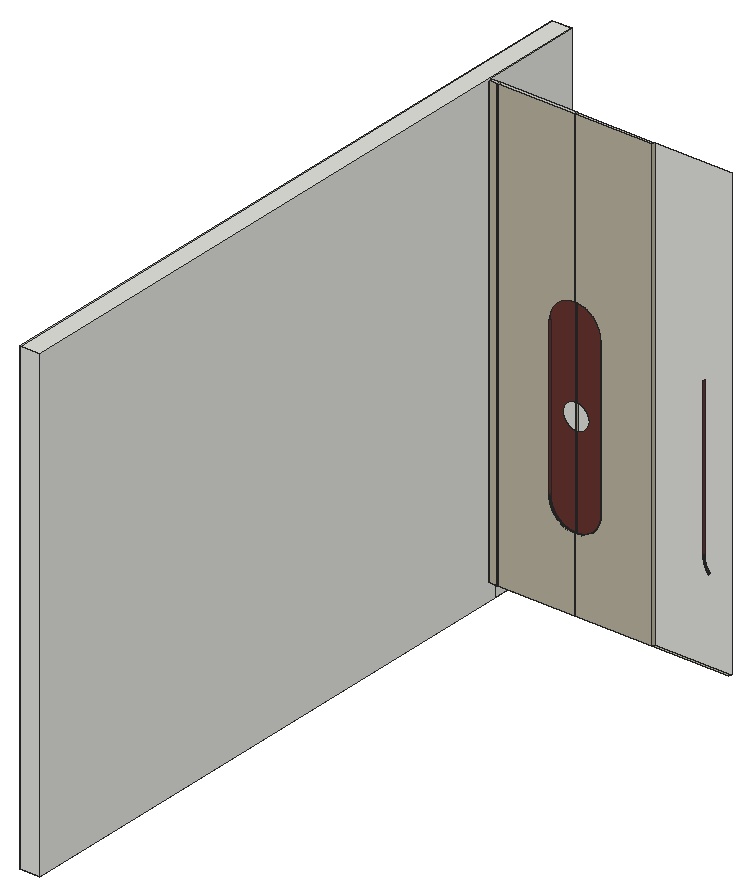
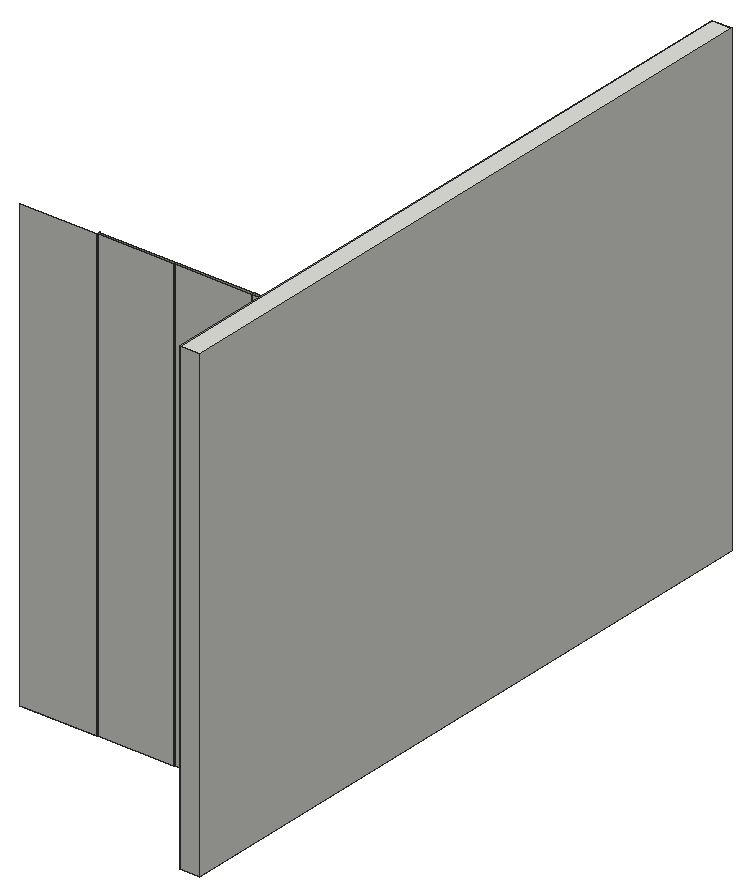
# SketchUp Ruby script. Lengths in millimetres.
U = 1.mm
M = Sketchup.active_model
def pt(a) = Geom::Point3d.new(a.map { |v| v * U })
def face(e, loops, mat)
  f = e.add_face(loops[0].map { |a| pt(a) })
  loops[1..].each { |l| e.add_face(l.map { |a| pt(a) }).erase! }
  f.material = f.back_material = mat if mat
  f
end
# faces: each face lists its corners as indices into pts; further lists are holes
def faces(e, pts, list, mat = nil) = list.each { |f| face(e, (f[0].is_a?(Array) ? f : [f]).map { |l| l.map { |i| pts[i] } }, mat) }
# xy, xz, yz: faces in a plane at the given z, y or x. An outline is a flat list of corners, or four numbers for a rectangle; further outlines are holes
def ring(l) = l.size == 4 ? [[l[0], l[1]], [l[2], l[1]], [l[2], l[3]], [l[0], l[3]]] : l.each_slice(2).to_a
def flat(e, list, mat, &to3) = list.each { |f| face(e, (f[0].is_a?(Array) ? f : [f]).map { |l| ring(l).map { |u, v| to3.(u, v) } }, mat) }
def xy(e, z, list, mat = nil) = flat(e, list, mat) { |x, y| [x, y, z] }
def xz(e, y, list, mat = nil) = flat(e, list, mat) { |x, z| [x, y, z] }
def yz(e, x, list, mat = nil) = flat(e, list, mat) { |y, z| [x, y, z] }
def lines(e, pts, list) = list.each { |a, b| e.add_line(pt(pts[a]), pt(pts[b])) }
# prism: a flat outline (further loops are holes) pulled along v
def prism(e, loops, v, mat = nil)
  f = face(e, loops, mat); d = Geom::Vector3d.new(v.map { |x| x * U })
  f.pushpull(f.normal.samedirection?(d) ? d.length : -d.length)
end
def box(e, o, s, mat = nil) = prism(e, [[o, [o[0] + s[0], o[1], o[2]], [o[0] + s[0], o[1] + s[1], o[2]], [o[0], o[1] + s[1], o[2]]]], [0, 0, s[2]], mat)
def at(x, y, z, deg = 0) = Geom::Transformation.translation(pt([x, y, z])) * Geom::Transformation.rotation(ORIGIN, Z_AXIS, deg.degrees)
def axes(o, x, y, z) = Geom::Transformation.new([*x, 0, *y, 0, *z, 0, *pt(o).to_a, 1])
def part(name) = M.definitions.add(name)
# library, detail: a bought-in or finely detailed component or shape, given as its bounding box
def library(name, o, s) = part(name).tap { |d| box(d.entities, o, s) }
def detail(e, o, s) = box(e.add_group.entities, o, s)
def put(e, d, t, mat = nil) = e.add_instance(d, t).tap { |i| i.material = mat if mat }
def group(e, t, mat = nil) = e.add_group.tap { |g| g.transformation = t; g.material = mat if mat }.entities
root = M.entities
M.materials.add("Uniboard-L17-Ambrette-4K").color = [104, 52, 49]
M.materials.add("Uniboard-L19-Putty-4K").color = [187, 181, 160]
xy(root,254,[[114.3,3403.6,165.1,3421.6],[168.1,3403.6,618.1,3421.6],[621.1,3403.6,1071,3421.6]])
xy(root,254,[[1074,3403.6,1524,3421.6]],"Uniboard-L19-Putty-4K")
xz(root,3403.6,[[114.3,254,165.1,2889.6],[168.1,254,618.1,254,618.1,685.8,616.3,685.9,611.5,686.1,606.7,686.5,602,687,597.2,687.7,592.5,688.5,587.8,689.5,583.2,690.6,578.5,691.9,574,693.3,569.4,694.8,565,696.5,560.5,698.3,556.2,700.3,551.9,702.4,547.6,704.7,543.5,707,539.4,709.5,535.4,712.2,531.5,714.9,527.7,717.8,523.9,720.8,520.3,723.9,516.7,727.1,513.3,730.4,506.7,737.4,503.6,741.1,500.6,744.8,497.8,748.6,495,752.5,492.4,756.5,489.9,760.6,487.5,764.8,485.3,769,483.2,773.3,481.2,777.7,479.4,782.1,477.7,786.6,476.1,791.1,474.7,795.7,473.5,800.3,472.3,805,471.4,809.6,470.5,814.4,469.9,819.1,469.3,823.9,469,828.6,468.7,833.4,468.7,1757.4,469,1762.2,469.3,1766.9,469.9,1771.7,470.5,1776.4,471.4,1781.2,472.3,1785.8,473.5,1790.5,474.7,1795.1,476.1,1799.7,477.7,1804.2,479.4,1808.7,481.2,1813.1,483.2,1817.5,485.3,1821.8,487.5,1826,489.9,1830.2,492.4,1834.3,495,1838.3,497.8,1842.2,500.6,1846,503.6,1849.7,506.7,1853.4,513.3,1860.4,516.7,1863.7,520.3,1866.9,523.9,1870,527.7,1873,531.5,1875.9,535.4,1878.6,539.4,1881.3,543.5,1883.8,547.6,1886.1,551.9,1888.4,556.2,1890.5,560.5,1892.5,565,1894.3,569.4,1896,574,1897.5,578.5,1898.9,583.2,1900.2,587.8,1901.3,592.5,1902.3,597.2,1903.1,602,1903.8,606.7,1904.3,611.5,1904.7,616.3,1904.9,618.1,1905,618.1,2889.6,168.1,2889.6],[621.1,254,1071,254,1071,2889.6,621.1,2889.6,621.1,1905,625.9,1904.9,630.6,1904.7,635.4,1904.3,640.2,1903.8,644.9,1903.1,649.6,1902.3,654.3,1901.3,659,1900.2,663.6,1898.9,668.2,1897.5,672.7,1896,677.2,1894.3,681.6,1892.5,686,1890.5,690.3,1888.4,694.5,1886.1,698.6,1883.8,702.7,1881.3,706.7,1878.6,710.6,1875.9,714.5,1873,718.2,1870,721.9,1866.9,725.4,1863.7,728.8,1860.4,732.2,1856.9,735.4,1853.4,738.5,1849.7,741.5,1846,744.4,1842.2,747.1,1838.3,749.7,1834.3,752.2,1830.2,754.6,1826,756.9,1821.8,759,1817.5,762.8,1808.7,764.5,1804.2,766,1799.7,767.4,1795.1,768.7,1790.5,769.8,1785.8,770.8,1781.2,771.6,1776.4,772.3,1771.7,772.8,1766.9,773.2,1762.2,773.4,1757.4,773.5,1752.6,773.5,838.2,773.4,833.4,773.2,828.6,772.8,823.9,772.3,819.1,771.6,814.4,770.8,809.6,769.8,805,768.7,800.3,767.4,795.7,766,791.1,764.5,786.6,762.8,782.1,759,773.3,756.9,769,754.6,764.8,752.2,760.6,749.7,756.5,747.1,752.5,744.4,748.6,741.5,744.8,738.5,741.1,735.4,737.4,732.2,733.9,728.8,730.4,725.4,727.1,721.9,723.9,718.2,720.8,714.5,717.8,710.6,714.9,706.7,712.2,702.7,709.5,698.6,707,694.5,704.7,690.3,702.4,686,700.3,681.6,698.3,677.2,696.5,672.7,694.8,668.2,693.3,663.6,691.9,659,690.6,654.3,689.5,649.6,688.5,644.9,687.7,640.2,687,635.4,686.5,630.6,686.1,625.9,685.9,621.1,685.8]],"Uniboard-L19-Putty-4K")
xz(root,3413.6,[[618.1,685.8,618.1,1217.7,617.1,1217.7,614.7,1217.9,612.3,1218,609.8,1218.3,604.4,1219.2,602.6,1219.6,600.2,1220.1,595.6,1221.5,593.2,1222.3,591,1223.2,588.7,1224.1,586.5,1225.1,582.1,1227.3,580,1228.5,577.9,1229.8,575.9,1231.1,573.9,1232.5,571.9,1234,570,1235.5,568.2,1237.1,564.6,1240.5,562.9,1242.2,561.3,1244,559.7,1245.9,556.7,1249.7,555.3,1251.7,554,1253.8,552.7,1255.8,551.5,1258,550.3,1260.1,548.3,1264.5,547.3,1266.8,545.7,1271.4,545,1273.7,544.3,1276.1,543.7,1278.5,543.2,1280.8,542.8,1283.2,542.5,1285.7,542.2,1288.1,542,1290.5,541.9,1293,541.9,1297.8,542,1300.3,542.2,1302.7,542.5,1305.1,542.8,1307.6,543.2,1310,543.7,1312.3,544.3,1314.7,545,1317.1,545.7,1319.4,547.3,1324,548.3,1326.3,550.3,1330.7,551.5,1332.8,552.7,1335,554,1337,555.3,1339.1,556.7,1341.1,559.7,1344.9,561.3,1346.8,562.9,1348.6,564.6,1350.3,568.2,1353.7,570,1355.3,571.9,1356.8,573.9,1358.3,575.9,1359.7,577.9,1361,580,1362.3,582.1,1363.5,586.5,1365.7,588.7,1366.7,591,1367.6,593.2,1368.5,595.6,1369.3,600.2,1370.7,602.6,1371.2,604.4,1371.6,609.8,1372.5,612.3,1372.8,614.7,1372.9,617.1,1373.1,618.1,1373.1,618.1,1905,616.3,1904.9,611.5,1904.7,606.7,1904.3,602,1903.8,597.2,1903.1,592.5,1902.3,587.8,1901.3,583.2,1900.2,578.5,1898.9,574,1897.5,569.4,1896,565,1894.3,560.5,1892.5,556.2,1890.5,551.9,1888.4,547.6,1886.1,543.5,1883.8,539.4,1881.3,535.4,1878.6,531.5,1875.9,527.7,1873,523.9,1870,520.3,1866.9,516.7,1863.7,513.3,1860.4,506.7,1853.4,503.6,1849.7,500.6,1846,497.8,1842.2,495,1838.3,492.4,1834.3,489.9,1830.2,487.5,1826,485.3,1821.8,483.2,1817.5,481.2,1813.1,479.4,1808.7,477.7,1804.2,476.1,1799.7,474.7,1795.1,473.5,1790.5,472.3,1785.8,471.4,1781.2,470.5,1776.4,469.9,1771.7,469.3,1766.9,469,1762.2,468.7,1757.4,468.7,833.4,469,828.6,469.3,823.9,469.9,819.1,470.5,814.4,471.4,809.6,472.3,805,473.5,800.3,474.7,795.7,476.1,791.1,477.7,786.6,479.4,782.1,481.2,777.7,483.2,773.3,485.3,769,487.5,764.8,489.9,760.6,492.4,756.5,495,752.5,497.8,748.6,500.6,744.8,503.6,741.1,506.7,737.4,513.3,730.4,516.7,727.1,520.3,723.9,523.9,720.8,527.7,717.8,531.5,714.9,535.4,712.2,539.4,709.5,543.5,707,547.6,704.7,551.9,702.4,556.2,700.3,560.5,698.3,565,696.5,569.4,694.8,574,693.3,578.5,691.9,583.2,690.6,587.8,689.5,592.5,688.5,597.2,687.7,602,687,606.7,686.5,611.5,686.1,616.3,685.9],[621.1,685.8,625.9,685.9,630.6,686.1,635.4,686.5,640.2,687,644.9,687.7,649.6,688.5,654.3,689.5,659,690.6,663.6,691.9,668.2,693.3,672.7,694.8,677.2,696.5,681.6,698.3,686,700.3,690.3,702.4,694.5,704.7,698.6,707,702.7,709.5,706.7,712.2,710.6,714.9,714.5,717.8,718.2,720.8,721.9,723.9,725.4,727.1,728.8,730.4,732.2,733.9,735.4,737.4,738.5,741.1,741.5,744.8,744.4,748.6,747.1,752.5,749.7,756.5,752.2,760.6,754.6,764.8,756.9,769,759,773.3,762.8,782.1,764.5,786.6,766,791.1,767.4,795.7,768.7,800.3,769.8,805,770.8,809.6,771.6,814.4,772.3,819.1,772.8,823.9,773.2,828.6,773.4,833.4,773.5,838.2,773.5,1752.6,773.4,1757.4,773.2,1762.2,772.8,1766.9,772.3,1771.7,771.6,1776.4,770.8,1781.2,769.8,1785.8,768.7,1790.5,767.4,1795.1,766,1799.7,764.5,1804.2,762.8,1808.7,759,1817.5,756.9,1821.8,754.6,1826,752.2,1830.2,749.7,1834.3,747.1,1838.3,744.4,1842.2,741.5,1846,738.5,1849.7,735.4,1853.4,732.2,1856.9,728.8,1860.4,725.4,1863.7,721.9,1866.9,718.2,1870,714.5,1873,710.6,1875.9,706.7,1878.6,702.7,1881.3,698.6,1883.8,694.5,1886.1,690.3,1888.4,686,1890.5,681.6,1892.5,677.2,1894.3,672.7,1896,668.2,1897.5,663.6,1898.9,659,1900.2,654.3,1901.3,649.6,1902.3,644.9,1903.1,640.2,1903.8,635.4,1904.3,630.6,1904.7,625.9,1904.9,621.1,1905,621.1,1373.1,622,1373.1,624.4,1372.9,626.9,1372.8,629.3,1372.5,634.7,1371.6,636.5,1371.2,638.9,1370.7,641.2,1370,643.6,1369.3,645.9,1368.5,648.2,1367.6,650.4,1366.7,652.6,1365.7,657,1363.5,659.1,1362.3,661.2,1361,663.2,1359.7,665.2,1358.3,667.2,1356.8,669.1,1355.3,671,1353.7,672.8,1352,676.2,1348.6,677.9,1346.8,679.4,1344.9,681,1343,682.4,1341.1,683.8,1339.1,685.2,1337,686.4,1335,687.7,1332.8,688.8,1330.7,689.9,1328.5,690.9,1326.3,692.7,1321.7,693.5,1319.4,694.2,1317.1,695.4,1312.3,695.9,1310,696.3,1307.6,696.7,1305.1,697.1,1300.3,697.2,1297.8,697.3,1295.4,697.2,1293,697.1,1290.5,696.7,1285.7,696.3,1283.2,695.9,1280.8,695.4,1278.5,694.2,1273.7,693.5,1271.4,692.7,1269.1,690.9,1264.5,689.9,1262.3,688.8,1260.1,687.7,1258,686.4,1255.8,685.2,1253.8,683.8,1251.7,682.4,1249.7,681,1247.8,679.4,1245.9,677.9,1244,676.2,1242.2,672.8,1238.8,671,1237.1,669.1,1235.5,667.2,1234,665.2,1232.5,663.2,1231.1,661.2,1229.8,659.1,1228.5,657,1227.3,652.6,1225.1,650.4,1224.1,648.2,1223.2,645.9,1222.3,643.6,1221.5,641.2,1220.8,638.9,1220.1,636.5,1219.6,634.7,1219.2,629.3,1218.3,626.9,1218,624.4,1217.9,622,1217.7,621.1,1217.7]],"Uniboard-L17-Ambrette-4K")
xz(root,3421.6,[[114.3,254,165.1,2889.6],[168.1,254,618.1,2889.6],[621.1,254,1071,2889.6],[1074,254,1524,2889.6]])
xz(root,3421.6,[[165.1,254,168.1,2889.6],[618.1,254,621.1,2889.6],[1071,254,1074,2889.6]],"Uniboard-L19-Putty-4K")
yz(root,114.3,[[3454.4,152.4,3454.4,254,3421.6,254,3421.6,2889.6,4013.2,2889.6,4013.2,152.4],[3403.6,254,3421.6,2889.6]])
yz(root,165.1,[[3403.6,254,3421.6,2889.6]],"Uniboard-L19-Putty-4K")
yz(root,168.1,[[3403.6,254,3421.6,2889.6]],"Uniboard-L19-Putty-4K")
yz(root,468.7,[[3403.6,833.4,3413.6,838.2],[3403.6,838.2,3413.6,1752.6]],"Uniboard-L17-Ambrette-4K")
yz(root,618.1,[[3403.6,254,3421.6,254,3421.6,2889.6,3403.6,2889.6,3403.6,1905,3413.6,1905,3413.6,685.8,3403.6,685.8]],"Uniboard-L19-Putty-4K")
yz(root,621.1,[[3403.6,254,3403.6,685.8,3413.6,685.8,3413.6,1905,3403.6,1905,3403.6,2889.6,3421.6,2889.6,3421.6,254]],"Uniboard-L19-Putty-4K")
yz(root,773.5,[[3403.6,838.2,3413.6,1752.6]],"Uniboard-L17-Ambrette-4K")
yz(root,1071,[[3403.6,254,3421.6,2889.6]],"Uniboard-L19-Putty-4K")
yz(root,1074,[[3403.6,254,3421.6,2889.6]],"Uniboard-L19-Putty-4K")
yz(root,1371.6,[[3403.6,838.2,3413.6,1752.6]],"Uniboard-L17-Ambrette-4K")
p = [[616.3,3403.6,685.9],[618.1,3403.6,685.8],[618.1,3413.6,685.8],[616.3,3413.6,685.9],[621.1,3403.6,685.8],[625.9,3403.6,685.9],
  [625.9,3413.6,685.9],[621.1,3413.6,685.8],[611.5,3403.6,686.1],[611.5,3413.6,686.1],[630.6,3403.6,686.1],[630.6,3413.6,686.1],
  [606.7,3403.6,686.5],[606.7,3413.6,686.5],[635.4,3403.6,686.5],[635.4,3413.6,686.5],[602,3403.6,687],[602,3413.6,687],
  [640.2,3403.6,687],[640.2,3413.6,687],[597.2,3403.6,687.7],[597.2,3413.6,687.7],[644.9,3403.6,687.7],[644.9,3413.6,687.7],
  [592.5,3403.6,688.5],[592.5,3413.6,688.5],[649.6,3403.6,688.5],[649.6,3413.6,688.5],[587.8,3403.6,689.5],[587.8,3413.6,689.5],
  [654.3,3403.6,689.5],[654.3,3413.6,689.5],[583.2,3403.6,690.6],[583.2,3413.6,690.6],[659,3403.6,690.6],[659,3413.6,690.6],
  [578.5,3403.6,691.9],[578.5,3413.6,691.9],[663.6,3403.6,691.9],[663.6,3413.6,691.9],[574,3403.6,693.3],[574,3413.6,693.3],
  [668.2,3403.6,693.3],[668.2,3413.6,693.3],[569.4,3403.6,694.8],[569.4,3413.6,694.8],[672.7,3403.6,694.8],[672.7,3413.6,694.8],
  [565,3403.6,696.5],[565,3413.6,696.5],[677.2,3403.6,696.5],[677.2,3413.6,696.5],[560.5,3403.6,698.3],[560.5,3413.6,698.3],
  [681.6,3403.6,698.3],[681.6,3413.6,698.3],[556.2,3403.6,700.3],[556.2,3413.6,700.3],[686,3403.6,700.3],[686,3413.6,700.3],
  [551.9,3403.6,702.4],[551.9,3413.6,702.4],[690.3,3403.6,702.4],[690.3,3413.6,702.4],[547.6,3403.6,704.7],[547.6,3413.6,704.7],
  [694.5,3403.6,704.7],[694.5,3413.6,704.7],[543.5,3403.6,707],[543.5,3413.6,707],[698.6,3403.6,707],[698.6,3413.6,707],
  [539.4,3403.6,709.5],[539.4,3413.6,709.5],[702.7,3403.6,709.5],[702.7,3413.6,709.5],[535.4,3403.6,712.2],[535.4,3413.6,712.2],
  [706.7,3403.6,712.2],[706.7,3413.6,712.2],[531.5,3403.6,714.9],[531.5,3413.6,714.9],[710.6,3403.6,714.9],[710.6,3413.6,714.9],
  [527.7,3403.6,717.8],[527.7,3413.6,717.8],[714.5,3403.6,717.8],[714.5,3413.6,717.8],[523.9,3403.6,720.8],[523.9,3413.6,720.8],
  [718.2,3403.6,720.8],[718.2,3413.6,720.8],[520.3,3403.6,723.9],[520.3,3413.6,723.9],[721.9,3403.6,723.9],[721.9,3413.6,723.9],
  [516.7,3403.6,727.1],[516.7,3413.6,727.1],[725.4,3403.6,727.1],[725.4,3413.6,727.1],[513.3,3403.6,730.4],[513.3,3413.6,730.4],
  [728.8,3403.6,730.4],[728.8,3413.6,730.4],[510,3403.6,733.9],[510,3413.6,733.9],[732.2,3403.6,733.9],[732.2,3413.6,733.9],
  [506.7,3403.6,737.4],[506.7,3413.6,737.4],[735.4,3403.6,737.4],[735.4,3413.6,737.4],[503.6,3403.6,741.1],[503.6,3413.6,741.1],
  [738.5,3403.6,741.1],[738.5,3413.6,741.1],[500.6,3403.6,744.8],[500.6,3413.6,744.8],[741.5,3403.6,744.8],[741.5,3413.6,744.8],
  [497.8,3403.6,748.6],[497.8,3413.6,748.6],[744.4,3403.6,748.6],[744.4,3413.6,748.6],[1400.7,3403.6,748.6],[1403.6,3403.6,744.8],
  [1403.6,3413.6,744.8],[1400.7,3413.6,748.6],[495,3403.6,752.5],[495,3413.6,752.5],[747.1,3403.6,752.5],[747.1,3413.6,752.5],
  [1398,3403.6,752.5],[1398,3413.6,752.5],[492.4,3403.6,756.5],[492.4,3413.6,756.5],[749.7,3403.6,756.5],[749.7,3413.6,756.5],
  [1395.3,3403.6,756.5],[1395.3,3413.6,756.5],[489.9,3403.6,760.6],[489.9,3413.6,760.6],[752.2,3403.6,760.6],[752.2,3413.6,760.6],
  [1392.8,3403.6,760.6],[1392.8,3413.6,760.6],[487.5,3403.6,764.8],[487.5,3413.6,764.8],[754.6,3403.6,764.8],[754.6,3413.6,764.8],
  [1390.5,3403.6,764.8],[1390.5,3413.6,764.8],[485.3,3403.6,769],[485.3,3413.6,769],[756.9,3403.6,769],[756.9,3413.6,769],
  [1388.2,3403.6,769],[1388.2,3413.6,769],[483.2,3403.6,773.3],[483.2,3413.6,773.3],[759,3403.6,773.3],[759,3413.6,773.3],
  [1386.1,3403.6,773.3],[1386.1,3413.6,773.3],[481.2,3403.6,777.7],[481.2,3413.6,777.7],[760.9,3403.6,777.7],[760.9,3413.6,777.7],
  [1384.1,3403.6,777.7],[1384.1,3413.6,777.7],[479.4,3403.6,782.1],[479.4,3413.6,782.1],[762.8,3403.6,782.1],[762.8,3413.6,782.1],
  [1382.3,3403.6,782.1],[1382.3,3413.6,782.1],[477.7,3403.6,786.6],[477.7,3413.6,786.6],[764.5,3403.6,786.6],[764.5,3413.6,786.6],
  [1380.6,3403.6,786.6],[1380.6,3413.6,786.6],[476.1,3403.6,791.1],[476.1,3413.6,791.1],[766,3403.6,791.1],[766,3413.6,791.1],
  [1379.1,3403.6,791.1],[1379.1,3413.6,791.1],[474.7,3403.6,795.7],[474.7,3413.6,795.7],[767.4,3403.6,795.7],[767.4,3413.6,795.7],
  [1377.7,3403.6,795.7],[1377.7,3413.6,795.7],[473.5,3403.6,800.3],[473.5,3413.6,800.3],[768.7,3403.6,800.3],[768.7,3413.6,800.3],
  [1376.4,3403.6,800.3],[1376.4,3413.6,800.3],[472.3,3403.6,805],[472.3,3413.6,805],[769.8,3403.6,805],[769.8,3413.6,805],
  [1375.3,3403.6,805],[1375.3,3413.6,805],[471.4,3403.6,809.6],[471.4,3413.6,809.6],[770.8,3403.6,809.6],[770.8,3413.6,809.6],
  [1374.3,3403.6,809.6],[1374.3,3413.6,809.6],[470.5,3403.6,814.4],[470.5,3413.6,814.4],[771.6,3403.6,814.4],[771.6,3413.6,814.4],
  [1373.5,3403.6,814.4],[1373.5,3413.6,814.4],[469.9,3403.6,819.1],[469.9,3413.6,819.1],[772.3,3403.6,819.1],[772.3,3413.6,819.1],
  [1372.8,3403.6,819.1],[1372.8,3413.6,819.1],[469.3,3403.6,823.9],[469.3,3413.6,823.9],[772.8,3403.6,823.9],[772.8,3413.6,823.9],
  [1372.3,3403.6,823.9],[1372.3,3413.6,823.9],[469,3403.6,828.6],[469,3413.6,828.6],[773.2,3403.6,828.6],[773.2,3413.6,828.6],
  [1371.9,3403.6,828.6],[1371.9,3413.6,828.6],[468.7,3403.6,833.4],[468.7,3413.6,833.4],[773.4,3403.6,833.4],[773.4,3413.6,833.4],
  [1371.7,3403.6,833.4],[1371.7,3413.6,833.4],[773.5,3403.6,838.2],[773.5,3413.6,838.2],[1371.6,3403.6,838.2],[1371.6,3413.6,838.2]]
faces(root,p,[[0,1,2,3],[4,5,6,7],[8,0,3,9],[5,10,11,6],[12,8,9,13],[10,14,15,11],[16,12,13,17],[14,18,19,15],
  [20,16,17,21],[18,22,23,19],[24,20,21,25],[22,26,27,23],[28,24,25,29],[26,30,31,27],[32,28,29,33],[30,34,35,31],
  [36,32,33,37],[34,38,39,35],[40,36,37,41],[38,42,43,39],[44,40,41,45],[42,46,47,43],[48,44,45,49],[46,50,51,47],
  [52,48,49,53],[50,54,55,51],[56,52,53,57],[54,58,59,55],[60,56,57,61],[58,62,63,59],[64,60,61,65],[62,66,67,63],
  [68,64,65,69],[66,70,71,67],[72,68,69,73],[70,74,75,71],[76,72,73,77],[74,78,79,75],[80,76,77,81],[78,82,83,79],
  [84,80,81,85],[82,86,87,83],[88,84,85,89],[86,90,91,87],[92,88,89,93],[90,94,95,91],[96,92,93,97],[94,98,99,95],
  [100,96,97,101],[98,102,103,99],[104,100,101,105],[102,106,107,103],[108,104,105,109],[106,110,111,107],[112,108,109,113],[110,114,115,111],
  [116,112,113,117],[114,118,119,115],[120,116,117,121],[118,122,123,119],[124,125,126,127],[128,120,121,129],[122,130,131,123],[132,124,127,133],
  [134,128,129,135],[130,136,137,131],[138,132,133,139],[140,134,135,141],[136,142,143,137],[144,138,139,145],[146,140,141,147],[142,148,149,143],
  [150,144,145,151],[152,146,147,153],[148,154,155,149],[156,150,151,157],[158,152,153,159],[154,160,161,155],[162,156,157,163],[164,158,159,165],
  [160,166,167,161],[168,162,163,169],[170,164,165,171],[166,172,173,167],[174,168,169,175],[176,170,171,177],[172,178,179,173],[180,174,175,181],
  [182,176,177,183],[178,184,185,179],[186,180,181,187],[188,182,183,189],[184,190,191,185],[192,186,187,193],[194,188,189,195],[190,196,197,191],
  [198,192,193,199],[200,194,195,201],[196,202,203,197],[204,198,199,205],[206,200,201,207],[202,208,209,203],[210,204,205,211],[212,206,207,213],
  [208,214,215,209],[216,210,211,217],[218,212,213,219],[214,220,221,215],[222,216,217,223],[224,218,219,225],[220,226,227,221],[228,222,223,229],
  [230,224,225,231],[226,232,233,227],[234,228,229,235],[236,230,231,237],[232,238,239,233],[240,234,235,241],[238,242,243,239],[244,240,241,245]],"Uniboard-L17-Ambrette-4K")
g1 = group(root,at(0,965.2,152.4))
box(g1,[0,-850.9,0],[114.3,3898.9,2743.2])
